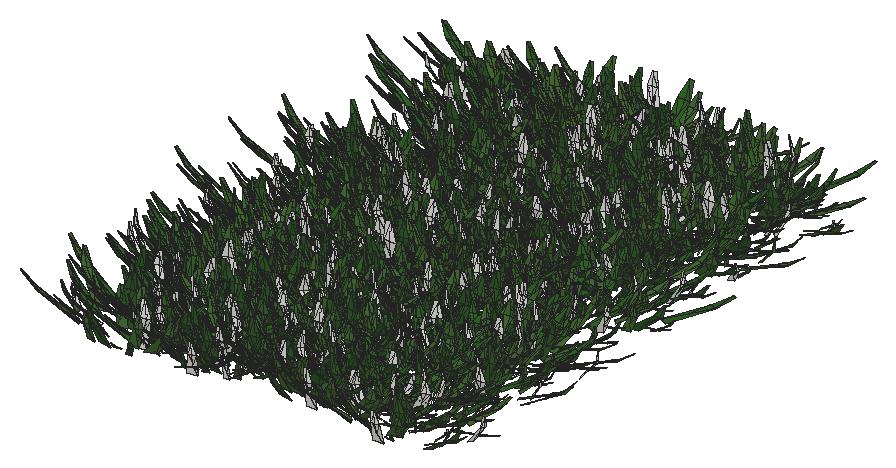
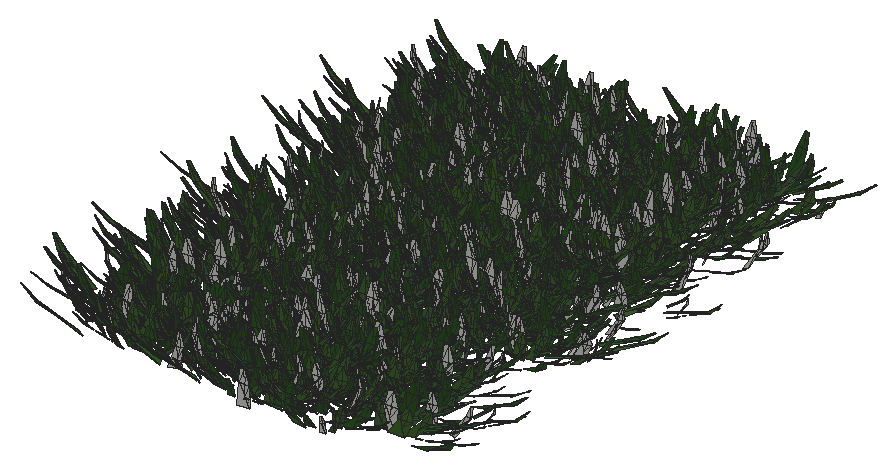
# SketchUp Ruby script. Lengths in inches.
U = 1.inch
M = Sketchup.active_model
def pt(a) = Geom::Point3d.new(a.map { |v| v * U })
def face(e, loops, mat)
  f = e.add_face(loops[0].map { |a| pt(a) })
  loops[1..].each { |l| e.add_face(l.map { |a| pt(a) }).erase! }
  f.material = f.back_material = mat if mat
  f
end
# faces: each face lists its corners as indices into pts; further lists are holes
def faces(e, pts, list, mat = nil) = list.each { |f| face(e, (f[0].is_a?(Array) ? f : [f]).map { |l| l.map { |i| pts[i] } }, mat) }
# xy, xz, yz: faces in a plane at the given z, y or x. An outline is a flat list of corners, or four numbers for a rectangle; further outlines are holes
def ring(l) = l.size == 4 ? [[l[0], l[1]], [l[2], l[1]], [l[2], l[3]], [l[0], l[3]]] : l.each_slice(2).to_a
def flat(e, list, mat, &to3) = list.each { |f| face(e, (f[0].is_a?(Array) ? f : [f]).map { |l| ring(l).map { |u, v| to3.(u, v) } }, mat) }
def xy(e, z, list, mat = nil) = flat(e, list, mat) { |x, y| [x, y, z] }
def xz(e, y, list, mat = nil) = flat(e, list, mat) { |x, z| [x, y, z] }
def yz(e, x, list, mat = nil) = flat(e, list, mat) { |y, z| [x, y, z] }
def lines(e, pts, list) = list.each { |a, b| e.add_line(pt(pts[a]), pt(pts[b])) }
# prism: a flat outline (further loops are holes) pulled along v
def prism(e, loops, v, mat = nil)
  f = face(e, loops, mat); d = Geom::Vector3d.new(v.map { |x| x * U })
  f.pushpull(f.normal.samedirection?(d) ? d.length : -d.length)
end
def box(e, o, s, mat = nil) = prism(e, [[o, [o[0] + s[0], o[1], o[2]], [o[0] + s[0], o[1] + s[1], o[2]], [o[0], o[1] + s[1], o[2]]]], [0, 0, s[2]], mat)
def at(x, y, z, deg = 0) = Geom::Transformation.translation(pt([x, y, z])) * Geom::Transformation.rotation(ORIGIN, Z_AXIS, deg.degrees)
def axes(o, x, y, z) = Geom::Transformation.new([*x, 0, *y, 0, *z, 0, *pt(o).to_a, 1])
def part(name) = M.definitions.add(name)
# library, detail: a bought-in or finely detailed component or shape, given as its bounding box
def library(name, o, s) = part(name).tap { |d| box(d.entities, o, s) }
def detail(e, o, s) = box(e.add_group.entities, o, s)
def put(e, d, t, mat = nil) = e.add_instance(d, t).tap { |i| i.material = mat if mat }
def group(e, t, mat = nil) = e.add_group.tap { |g| g.transformation = t; g.material = mat if mat }.entities
root = M.entities
M.materials.add("Material82").color = [68, 110, 58]
M.materials.add("Material83").color = [48, 90, 38]
M.materials.add("Material84").color = [68, 110, 48]
M.materials.add("Material85").color = [48, 90, 48]
M.materials.add("Material86").color = [58, 110, 58]
M.materials.add("Material87").color = [58, 90, 38]
M.materials.add("Material88").color = [68, 100, 58]
M.materials.add("Material89").color = [48, 100, 38]
c1 = part("grass00")
p = [[-0.6875,0.15,0],[-0.56,0.08,5.52],[-0.04,0.03,2.76],[0.48,-0.02,0],[0.35,-0.02,5.52],[-0.1,-0.14,5.52],
  [-0.12,0.65,8.37],[-0.42,0.65,8.37]]
faces(c1.entities,p,[[0,1,2,3],[3,2,4],[1,5,2],[5,4,2],[1,6,5],[4,5,6],[7,6,1]])
c2 = part("Group16\#1")
put(c2.entities,c1,axes([1.44,-0.61,-0.01],[0.05352,0.12609,0],[-0.10704,0.04543,0.07239],[0.06664,-0.02828,0.11628]),"Material85")
put(c2.entities,c1,axes([0.76,-0.15,-0.01],[0.04676,0.24062,0],[-0.23162,0.04501,0.06642],[0.0652,-0.01267,0.23595]),"Material82")
put(c2.entities,c1,axes([0.79,0.01,-0.01],[-0.00606,0.34651,0],[-0.34381,-0.00602,0.0432],[0.04319,0.00076,0.34386]))
put(c2.entities,c1,axes([1,0.23,-0.01],[-0.07192,0.31144,0],[-0.28722,-0.06632,0.1236],[0.12043,0.02781,0.29478]),"Material84")
put(c2.entities,c1,axes([1.66,0.77,-0.01],[-0.13828,0.29651,0],[-0.21551,-0.1005,0.22471],[0.20365,0.09498,0.23779]),"Material89")
put(c2.entities,c1,axes([0.6875,0.52,-0.01],[-0.18126,0.24051,0],[-0.22746,-0.17142,0.09788],[0.07817,0.05891,0.28481]),"Material84")
put(c2.entities,c1,axes([0.68,0.78,-0.01],[-0.215,0.18688,0],[-0.12385,-0.14248,0.21334],[0.13995,0.16101,0.18878]),"Material82")
put(c2.entities,c1,axes([0.56,1,-0.01],[-0.13756,0.07624,0],[-0.06159,-0.11112,0.0927],[0.04494,0.08108,0.12705]),"Material84")
put(c2.entities,c1,axes([0.2,0.64,-0.01],[-0.23729,0.07254,0],[-0.05711,-0.18681,0.153],[0.04473,0.14632,0.19535]),"Material89")
put(c2.entities,c1,axes([0.0625,0.72,-0.01],[-0.28874,0.02525,0],[-0.02179,-0.24916,0.14647],[0.01276,0.14591,0.25012]),"Material82")
put(c2.entities,c1,axes([-0.08,0.62,-0.01],[-0.34089,-0.04187,0],[0.03255,-0.26504,0.216],[-0.02633,0.21439,0.26703]),"Material89")
put(c2.entities,c1,axes([-0.34,0.98,-0.01],[-0.14314,-0.0493,0],[0.04397,-0.12769,0.06843],[-0.02228,0.0647,0.13505]),"Material89")
put(c2.entities,c1,axes([-0.87,1.45,-0.01],[-0.23488,-0.14114,0],[0.13761,-0.22901,0.06087],[-0.03135,0.05217,0.26717]))
put(c2.entities,c1,axes([-0.72,0.77,-0.01],[-0.14208,-0.13251,0],[0.07209,-0.0773,0.16301],[-0.11118,0.11922,0.1057]),"Material89")
put(c2.entities,c1,axes([-0.62,0.43,-0.01],[-0.14845,-0.21203,0],[0.18654,-0.13061,0.12304],[-0.10079,0.07057,0.22772]),"Material82")
put(c2.entities,c1,axes([-0.68,0.29,-0.01],[-0.13639,-0.32136,0],[0.31723,-0.13464,0.05579],[-0.05136,0.0218,0.34462]),"Material83")
put(c2.entities,c1,axes([-0.64,0.125,-0.01],[-0.0458,-0.23569,0],[0.22124,-0.043,0.08276],[-0.08124,0.01579,0.22538]),"Material86")
put(c2.entities,c1,axes([-1.6,-0.03,-0.01],[0.00576,-0.32897,0],[0.27526,0.00482,0.18018],[-0.18015,-0.00315,0.2753]),"Material84")
put(c2.entities,c1,axes([-1.36,-0.31,-0.01],[0.05718,-0.24765,0],[0.18172,0.04196,0.17267],[-0.16825,-0.03885,0.1865]),"Material89")
put(c2.entities,c1,axes([-1.54,-0.72,-0.01],[0.06537,-0.14017,0],[0.13555,0.06321,0.03939],[-0.0357,-0.01665,0.14956]))
put(c2.entities,c1,axes([-1.19,-0.9,-0.01],[0.09597,-0.12735,0],[0.11214,0.08451,0.07557],[-0.06035,-0.04548,0.14042]),"Material88")
put(c2.entities,c1,axes([-0.47,-0.54,-0.01],[0.11588,-0.10072,0],[0.0618,0.0711,0.12124],[-0.07953,-0.0915,0.0942]))
put(c2.entities,c1,axes([-0.47,-0.84,-0.01],[0.11927,-0.0661,0],[0.06603,0.11913,0.00646],[-0.00313,-0.00565,0.13621]),"Material84")
put(c2.entities,c1,axes([-0.38,-1.24,-0.01],[0.28037,-0.08571,0],[0.0618,0.20215,0.20315],[-0.05939,-0.19428,0.21139]),"Material88")
put(c2.entities,c1,axes([-0.06,-0.66,-0.01],[0.22719,-0.01987,0],[0.01247,0.14255,0.17758],[-0.01547,-0.17691,0.1431]),"Material87")
put(c2.entities,c1,axes([0.11,-0.89,-0.01],[0.14882,0.01828,0],[-0.01058,0.08611,0.12229],[0.01491,-0.12138,0.08676]),"Material85")
put(c2.entities,c1,axes([0.25,-0.72,-0.01],[0.20481,0.07053,0],[-0.06206,0.18022,0.10291],[0.03351,-0.0973,0.1906]),"Material85")
put(c2.entities,c1,axes([0.85,-1.42,-0.01],[0.16481,0.09904,0],[-0.09472,0.15762,0.05616],[0.02893,-0.04814,0.18389]),"Material84")
put(c2.entities,c1,axes([1.01,-1.09,-0.01],[0.21858,0.20385,0],[-0.17495,0.1876,0.15339],[0.10462,-0.11218,0.25652]),"Material89")
put(c2.entities,c1,axes([1.01,-0.71,-0.01],[0.08733,0.12473,0],[-0.06445,0.04512,0.13037],[0.1068,-0.07477,0.07867]),"Material85")
c3 = part("Group15\#1")
put(c3.entities,c2,at(0,0,0))
c4 = part("3darcstudiotree_grass00\#1")
put(c4.entities,c3,at(0,0,0))
put(root,c4,axes([1826.71,976.55,-29.74],[-0.54088,1.62044,0],[-3.31155,-0.17191,-0.03263],[-0.19335,-0.01004,1.49628]))
put(root,c4,axes([1826.9,975.01,-29.74],[3.70566,-0.42814,0],[1.15173,1.5504,-0.01036],[0.01836,0.02471,1.93559]))
put(root,c4,axes([1827.4,940.33,-29.74],[2.92691,-1.3802,0],[3.11862,1.02859,-0.02296],[0.10607,0.03499,1.8355]))
put(root,c4,axes([1827.2,994.31,-29.74],[-0.97344,1.33602,0],[-4.5066,-0.51069,-0.06106],[-0.24596,-0.02787,1.47293]))
put(root,c4,axes([1827.02,963.53,-29.74],[4.64499,-0.27977,0],[0.53132,1.372,-0.02943],[0.02555,0.06597,1.51666]))
put(root,c4,axes([1828.48,961.14,-29.74],[-0.18207,-1.50592,0],[4.09357,-0.07698,-0.05646],[0.28834,-0.00542,1.57058]))
put(root,c4,axes([1827.15,950.76,-29.74],[2.47814,1.17598,0],[-3.14029,1.02922,-0.05468],[-0.21842,0.07159,1.58958]))
put(root,c4,axes([1827.12,973.05,-29.74],[4.42055,0.62646,0],[-1.4719,1.61538,-0.03831],[-0.06085,0.06679,1.53223]))
put(root,c4,axes([1827.64,989.9,-29.74],[4.51641,-0.1704,0],[0.33815,1.39393,-0.00501],[0.00291,0.012,1.62495]))
put(root,c4,axes([1827.34,952.9375,-29.74],[2.33395,1.59128,0],[-3.69314,0.84246,-0.02506],[-0.12399,0.02828,1.82822]))
put(root,c4,axes([1827.93,944.71,-29.74],[3.72841,-0.11021,0],[0.34874,1.83494,-0.00347],[0.00143,0.00753,1.92949]))
put(root,c4,axes([1828.92,986.01,-29.74],[-2.15234,1.14546,0],[-3.3995,-0.99347,-0.05517],[-0.2418,-0.07066,1.72999]))
put(root,c4,axes([1828.23,959.73,-29.74],[2.3917,1.38211,0],[-2.775,0.74686,-0.01403],[-0.09111,0.02452,1.97952]))
put(root,c4,axes([1828.32,968.4,-29.74],[3.05644,0.96272,0],[-2.54771,1.25799,-0.04015],[-0.1144,0.05649,1.39698]))
put(root,c4,axes([1828.88,955.42,-29.74],[0.44258,1.4547,0],[-3.4051,0.16112,-0.01784],[-0.12417,0.00588,1.80168]))
put(root,c4,axes([1830.52,982.97,-29.74],[-1.45799,-1.43911,0],[3.11235,-0.49041,-0.01431],[0.09188,-0.01448,1.73701]))
put(root,c4,axes([1830.67,942.56,-29.74],[-2.77273,1.25915,0],[-2.61353,-0.89509,-0.01448],[-0.05898,-0.0202,1.39954]))
put(root,c4,axes([1831.64,944.09,-29.74],[-3.67224,-0.62774,0],[1.3268,-1.20717,-0.04544],[0.10775,-0.09803,1.4908]))
put(root,c4,axes([1831.89,976.69,-29.74],[-4.47177,0.4092,0],[-0.80597,-1.36984,-0.03599],[-0.04373,-0.07433,1.43677]))
put(root,c4,axes([1831.27,954.99,-29.74],[-3.07968,1.30519,0],[-3.32937,-1.22181,-0.01383],[-0.04412,-0.01619,1.48532]))
put(root,c4,axes([1830.8125,966.41,-29.74],[3.91717,0.58785,0],[-1.40512,1.45623,-0.01203],[-0.02325,0.0241,1.60927]))
put(root,c4,axes([1832.68,961.55,-29.74],[-1.04981,-1.26066,0],[3.51989,-0.45588,-0.02104],[0.10484,-0.01358,1.45661]))
put(root,c4,axes([1831.94,958.11,-29.74],[3.15172,-0.92963,0],[2.70365,1.42561,-0.02614],[0.06865,0.0362,1.48366]))
put(root,c4,axes([1832.72,964.35,-29.74],[-4.56421,0.17831,0],[-0.33265,-1.32435,-0.0174],[-0.0117,-0.04658,1.72585]))
put(root,c4,axes([1833.2,990.04,-29.74],[-3.08784,-0.53374,0],[1.78756,-1.6084,-0.00176],[0.00414,-0.00372,1.95594]))
put(root,c4,axes([1832.26,950.46,-29.74],[-2.14552,1.35971,0],[-3.80804,-0.93454,-0.04897],[-0.2422,-0.05944,1.9584]))
put(root,c4,axes([1831.72,947.17,-29.74],[3.03533,0.518,0],[-1.31858,1.2017,-0.02703],[-0.08286,0.07551,1.9211]))
put(root,c4,axes([1833.56,972.37,-29.74],[-2.79081,-0.68685,0],[2.20267,-1.39196,-0.00523],[0.01654,-0.01045,1.86317]))
put(root,c4,axes([1833.69,975.79,-29.74],[-3.42781,-0.73376,0],[1.91044,-1.38806,-0.04387],[0.11882,-0.08633,1.70431]))
put(root,c4,axes([1833,948.51,-29.74],[-3.41152,0.77464,0],[-2.34689,-1.60751,-0.0199],[-0.0471,-0.03226,1.67187]))
put(root,c4,axes([1832.01,971.16,-29.74],[1.53269,1.16919,0],[-3.90157,0.79546,-0.03477],[-0.15934,0.03249,1.69826]))
put(root,c4,axes([1833.29,959.12,-29.74],[-2.82754,1.11661,0],[-2.90837,-1.14544,-0.05526],[-0.21558,-0.0849,1.69871]))
put(root,c4,axes([1833.3,952.53,-29.74],[2.39859,-1.38317,0],[2.89597,0.78107,-0.02882],[0.1286,0.03468,1.42183]))
put(root,c4,axes([1833.73,996.9375,-29.74],[0.37671,-1.60669,0],[3.58296,0.13066,-0.04487],[0.23434,0.00855,1.41449]))
put(root,c4,axes([1834.14,995.4375,-29.74],[-4.41181,-0.09171,0],[0.23476,-1.75641,-0.0488],[0.01273,-0.09527,1.65721]))
put(root,c4,axes([1834,940.76,-29.74],[-3.47293,0.19496,0],[-0.50842,-1.40863,-0.03826],[-0.03299,-0.09141,1.65468]))
put(root,c4,axes([1834.5625,991.8,-29.74],[-4.2727,-0.29638,0],[0.78575,-1.76178,-0.04722],[0.03378,-0.07573,1.40384]))
put(root,c4,axes([1833.22,987.32,-29.74],[-0.9668,1.66725,0],[-3.92404,-0.3539,-0.0233],[-0.11915,-0.01075,1.58282]))
put(root,c4,axes([1833.27,968.64,-29.74],[3.78841,0.96012,0],[-2.55963,1.5708,-0.03131],[-0.07104,0.04359,1.48921]))
put(root,c4,axes([1833.51,981.64,-29.74],[2.7139,1.45109,0],[-3.63417,1.0571,-0.05484],[-0.17137,0.04985,1.31443]))
put(root,c4,axes([1834.07,979.63,-29.74],[3.41186,0.04199,0],[-0.11049,1.39641,-0.01718],[-0.0038,0.04797,1.88076]))
put(root,c4,axes([1836.15,958.1,-29.74],[-3.09292,-0.92086,0],[2.57207,-1.3436,-0.01411],[0.04505,-0.02353,1.69584]))
put(root,c4,axes([1834.3,985.4,-29.74],[0.1551,1.54916,0],[-4.73746,0.07377,-0.04149],[-0.18002,0.0028,1.54325]))
put(root,c4,axes([1836.33,976.88,-29.74],[0.67498,-1.80639,0],[4.18251,0.24307,-0.00777],[0.03281,0.00191,1.3523]))
put(root,c4,axes([1836.49,972.86,-29.74],[-0.75947,-1.30953,0],[4.19896,-0.37875,-0.04627],[0.26037,-0.02349,1.86363]))
put(root,c4,axes([1836.53,959.17,-29.74],[-4.1346,0.13575,0],[-0.2838,-1.34436,-0.02559],[-0.01617,-0.0766,1.95328]))
put(root,c4,axes([1837.31,970.48,-29.74],[1.00092,-1.32759,0],[4.42574,0.51896,-0.06029],[0.29852,0.035,1.78762]))
put(root,c4,axes([1837,991.66,-29.74],[2.10537,-1.23806,0],[3.71835,0.98344,-0.05795],[0.27877,0.07373,1.94389]))
put(root,c4,axes([1836.35,946.54,-29.74],[3.79547,0.16316,0],[-0.37027,1.33962,-0.03498],[-0.02197,0.07948,1.48455]))
put(root,c4,axes([1837.2,966.05,-29.74],[-3.00276,0.99555,0],[-2.11915,-0.9941,-0.00081],[-0.00373,-0.00175,1.76997]))
put(root,c4,axes([1838.32,984.25,-29.74],[-0.04764,-1.42757,0],[4.50476,-0.02338,-0.00745],[0.04284,-0.00022,1.94284]))
put(root,c4,axes([1837.01,942.28,-29.74],[0.27257,1.5962,0],[-3.57048,0.09483,-0.04154],[-0.28788,0.00765,1.86323]))
put(root,c4,axes([1838.46,979.48,-29.74],[-4.51182,-0.35471,0],[0.87439,-1.72977,-0.01918],[0.02129,-0.04212,1.90358]))
put(root,c4,axes([1837.23,986.4375,-29.74],[2.9902,-0.77103,0],[1.83544,1.10708,-0.045],[0.13449,0.08112,1.37282]))
put(root,c4,axes([1838.51,964.39,-29.74],[0.52861,-1.48035,0],[4.44113,0.24665,-0.00524],[0.03043,0.00169,1.97007]))
put(root,c4,axes([1836.8,953.83,-29.74],[1.62026,1.14881,0],[-2.90984,0.63829,-0.00131],[-0.00892,0.00196,1.9458]))
put(root,c4,axes([1837.83,944.28,-29.74],[-3.07094,0.93295,0],[-2.23562,-1.14452,-0.00087],[-0.00325,-0.00166,1.68429]))
put(root,c4,axes([1838.87,950.63,-29.74],[-1.32818,-1.26932,0],[4.11875,-0.67029,-0.01762],[0.07227,-0.01176,1.48208]))
put(root,c4,axes([1836.96,948.25,-29.74],[3.48613,0.95688,0],[-2.23612,1.26704,-0.01513],[-0.04219,0.02391,1.43215]))
put(root,c4,axes([1838.05,981.34,-29.74],[3.73229,-0.67208,0],[1.78653,1.54305,-0.05401],[0.10032,0.08665,1.44188]))
put(root,c4,axes([1839.69,994.4375,-29.74],[-3.64932,-0.7532,0],[1.94147,-1.463,-0.05348],[0.14522,-0.10943,1.83786]))
put(root,c4,axes([1838.4,968.61,-29.74],[4.39358,-0.14103,0],[0.35283,1.70956,-0.02372],[0.00876,0.04243,1.48337]))
put(root,c4,axes([1839.88,996.02,-29.74],[-4.22243,0.41861,0],[-0.86072,-1.35028,-0.03206],[-0.04838,-0.0759,1.63785]))
put(root,c4,axes([1838.9,987.81,-29.74],[2.4549,0.99675,0],[-3.14112,1.20322,-0.03466],[-0.14383,0.05509,1.89896]))
put(root,c4,axes([1838.95,974.69,-29.74],[3.48474,0.89145,0],[-2.45497,1.49256,-0.05832],[-0.13986,0.08503,1.48992]))
put(root,c4,axes([1839.48,990.48,-29.74],[-0.03901,1.43427,0],[-3.74587,-0.01585,-0.03184],[-0.19446,-0.00082,1.71482]))
put(root,c4,axes([1839.86,962.16,-29.74],[-1.95042,1.47202,0],[-4.16072,-0.85742,-0.06253],[-0.2988,-0.06158,1.89715]))
put(root,c4,axes([1839.76,955.55,-29.74],[3.54296,-0.10072,0],[0.24357,1.33252,-0.00836],[0.00467,0.02557,1.97523]))
put(root,c4,axes([1841.96,972.91,-29.74],[-3.58618,-0.76762,0],[2.12856,-1.54662,-0.04044],[0.10752,-0.07813,1.86421]))
put(root,c4,axes([1842.24,968.36,-29.74],[-3.71376,-0.4791,0],[1.06109,-1.27925,-0.035],[0.07367,-0.08882,1.73222]))
put(root,c4,axes([1842.79,988.51,-29.74],[-3.76687,-0.82913,0],[2.27178,-1.60524,-0.0179],[0.04066,-0.02873,1.62858]))
put(root,c4,axes([1841.95,950.84,-29.74],[-3.28554,0.84585,0],[-2.43757,-1.4726,-0.04574],[-0.1384,-0.08361,1.85022]))
put(root,c4,axes([1842.7,949.5,-29.74],[0.43132,-1.66774,0],[3.95027,0.1589,-0.00761],[0.04938,0.00199,1.94156]))
put(root,c4,axes([1842.96,976.58,-29.74],[-3.03865,-1.23581,0],[2.76731,-1.05827,-0.04714],[0.18592,-0.0711,1.58733]))
put(root,c4,axes([1841.55,945.875,-29.74],[4.71636,-0.1967,0],[0.48906,1.82382,-0.02611],[0.01545,0.05763,1.96192]))
put(root,c4,axes([1842.64,979.12,-29.74],[-3.07129,1.23004,0],[-2.90171,-1.12685,-0.02428],[-0.07533,-0.02925,1.32917]))
put(root,c4,axes([1843.55,953.86,-29.74],[-3.14124,-0.52931,0],[1.80451,-1.66556,-0.04539],[0.09971,-0.09203,1.92461]))
put(root,c4,axes([1842.27,997.4,-29.74],[4.37264,-0.16186,0],[0.38997,1.63854,-0.03728],[0.02119,0.08905,1.90298]))
put(root,c4,axes([1842.62,991.83,-29.74],[4.22982,-0.69798,0],[1.45654,1.37281,-0.04818],[0.09708,0.0915,1.47658]))
put(root,c4,axes([1842.875,990.87,-29.74],[3.5272,-0.10967,0],[0.36977,1.84972,-0.03935],[0.01267,0.0634,1.44542]))
put(root,c4,axes([1843.61,983.14,-29.74],[2.22522,-0.98382,0],[3.26699,1.14926,-0.04874],[0.15967,0.05617,1.44038]))
put(root,c4,axes([1842.81,957.58,-29.74],[4.40761,-0.00182,0],[0.00468,1.76466,-0.04894],[0.00022,0.08123,1.41164]))
put(root,c4,axes([1844.71,975.77,-29.74],[-3.1255,-0.93872,0],[2.35839,-1.22127,-0.01582],[0.04515,-0.02338,1.37394]))
put(root,c4,axes([1843.66,971.33,-29.74],[-2.15998,1.50569,0],[-3.5128,-0.78375,-0.02589],[-0.10439,-0.02329,1.40149]))
put(root,c4,axes([1844.14,994.6875,-29.74],[2.50422,-1.12718,0],[2.64209,0.91293,-0.00209],[0.0092,0.00318,1.54397]))
put(root,c4,axes([1844.3,986.33,-29.74],[-3.79899,1.04858,0],[-2.13311,-1.20197,-0.01309],[-0.05055,-0.02848,1.87779]))
put(root,c4,axes([1844.97,956.11,-29.74],[-0.77442,-1.59147,0],[3.42237,-0.25901,-0.00431],[0.02185,-0.00165,1.34772]))
put(root,c4,axes([1845.25,942.86,-29.74],[-1.56215,-1.16443,0],[3.47638,-0.72535,-0.0302],[0.1517,-0.03165,1.67548]))
put(root,c4,axes([1845.33,961.6,-29.74],[0.16922,-1.40325,0],[3.56749,0.06691,-0.0123],[0.08099,0.00152,1.7643]))
put(root,c4,axes([1844.16,965.91,-29.74],[3.21803,0.34517,0],[-1.06694,1.54707,-0.02379],[-0.03071,0.04453,1.49895]))
put(root,c4,axes([1843.92,959.62,-29.74],[1.18275,1.22871,0],[-4.35683,0.65227,-0.02635],[-0.11985,0.01794,1.69955]))
put(root,c4,axes([1845.58,981.5,-29.74],[-4.55654,0.30056,0],[-0.72952,-1.72007,-0.00717],[-0.00538,-0.01268,1.50735]))
put(root,c4,axes([1845.07,964.58,-29.74],[2.66801,-0.76193,0],[2.24823,1.2244,-0.04376],[0.15596,0.08494,1.7457]))
put(root,c4,axes([1847.17,972.15,-29.74],[-2.4386,-1.43306,0],[3.07254,-0.81318,-0.00883],[0.05033,-0.01332,1.90461]))
put(root,c4,axes([1847.54,990.58,-29.74],[-2.69612,-1.17454,0],[3.29179,-1.17522,-0.01753],[0.05781,-0.02064,1.48083]))
put(root,c4,axes([1845.5,944.46,-29.74],[-0.169,1.77802,0],[-4.32571,-0.06395,-0.00219],[-0.00941,-0.00014,1.39308]))
put(root,c4,axes([1847.73,948.11,-29.74],[-3.83813,-1.06248,0],[2.06139,-1.15817,-0.02484],[0.08815,-0.04953,1.66133]))
put(root,c4,axes([1847.43,984.43,-29.74],[-4.08007,0.11151,0],[-0.22831,-1.29918,-0.01842],[-0.00694,-0.03947,1.34789]))
put(root,c4,axes([1847.91,942.67,-29.74],[-3.13096,0.65051,0],[-1.62991,-1.22011,-0.01732],[-0.0588,-0.04402,1.90951]))
put(root,c4,axes([1849.12,995.01,-29.74],[-1.34356,-1.54381,0],[4.22745,-0.57221,-0.00214],[0.01038,-0.00141,1.72072]))
put(root,c4,axes([1847.18,950.22,-29.74],[3.83567,0.80348,0],[-1.71741,1.27513,-0.04207],[-0.13622,0.10114,1.89419]))
put(root,c4,axes([1847.6,966.3125,-29.74],[2.14752,1.24419,0],[-2.84206,0.76295,-0.02533],[-0.12904,0.03464,1.58831]))
put(root,c4,axes([1848.2,988.64,-29.74],[4.00755,-0.76372,0],[1.77132,1.44561,-0.00312],[0.00773,0.00631,1.73901]))
put(root,c4,axes([1847.9,959.82,-29.74],[0.92286,1.78615,0],[-4.03148,0.32396,-0.0503],[-0.25163,0.02022,1.57458]))
put(root,c4,axes([1848.24,974.88,-29.74],[-1.5079,1.48015,0],[-3.78766,-0.60014,-0.02547],[-0.10708,-0.01697,1.38631]))
put(root,c4,axes([1849.28,956.86,-29.74],[0.88426,-1.72062,0],[4.38154,0.35021,-0.041],[0.21175,0.01693,1.76588]))
put(root,c4,axes([1848.11,952.75,-29.74],[4.1439,0.48612,0],[-1.21296,1.60815,-0.03162],[-0.038,0.05038,1.3441]))
put(root,c4,axes([1847.97,967.88,-29.74],[2.12924,1.06786,0],[-3.55371,1.10206,-0.01217],[-0.05143,0.01595,1.82194]))
put(root,c4,axes([1849.54,943.78,-29.74],[1.5808,-1.43275,0],[3.65536,0.62726,-0.04597],[0.19603,0.03364,1.38947]))
put(root,c4,axes([1850.43,947.09,-29.74],[-4.27451,-0.64112,0],[1.27307,-1.32012,-0.04106],[0.09351,-0.09696,1.71966]))
put(root,c4,axes([1850.35,992.01,-29.74],[-3.75297,0.08152,0],[-0.23562,-1.68719,-0.02509],[-0.00578,-0.04142,1.34616]))
put(root,c4,axes([1851,982.35,-29.74],[-0.74737,-1.75822,0],[4.00395,-0.2647,-0.02808],[0.1526,-0.01009,1.67665]))
put(root,c4,axes([1850.24,963.58,-29.74],[2.37533,-1.57622,0],[3.03149,0.71052,-0.0411],[0.20378,0.04776,1.52451]))
put(root,c4,axes([1849.44,977.06,-29.74],[3.22242,0.46316,0],[-1.61234,1.7447,-0.03532],[-0.06153,0.06658,1.79519]))
put(root,c4,axes([1849.93,971.43,-29.74],[0.53134,1.4221,0],[-3.42638,0.19911,-0.04131],[-0.21204,0.01232,1.34689]))
put(root,c4,axes([1850.41,962.64,-29.74],[3.9417,-1.03975,0],[1.84996,1.09076,-0.03191],[0.12762,0.07525,1.79443]))
put(root,c4,axes([1850.8,955.36,-29.74],[3.56947,-0.45549,0],[1.31887,1.60745,-0.01717],[0.02449,0.02985,1.48777]))
put(root,c4,axes([1850.88,978.75,-29.74],[0.55525,1.71346,0],[-3.482,0.17549,-0.04145],[-0.30813,0.01553,1.97198]))
put(root,c4,axes([1850.63,985.74,-29.74],[3.66484,0.89609,0],[-2.00603,1.27601,-0.03504],[-0.12347,0.07854,1.90819]))
put(root,c4,axes([1852.84,948.68,-29.74],[-1.10349,-1.4395,0],[4.41957,-0.52692,-0.03772],[0.14279,-0.01702,1.36861]))
put(root,c4,axes([1852.64,978.59,-29.74],[-2.20687,1.14075,0],[-3.09016,-0.92978,-0.05103],[-0.23957,-0.07208,1.72023]))
put(root,c4,axes([1853.1,990.62,-29.74],[-3.32366,1.12138,0],[-2.70082,-1.24501,-0.05065],[-0.15287,-0.07047,1.44592]))
put(root,c4,axes([1854.1875,975.37,-29.74],[-2.7638,-1.30283,0],[3.13183,-1.03331,-0.01878],[0.07913,-0.02611,1.68146]))
put(root,c4,axes([1854.41,968.09,-29.74],[-3.16827,-0.67396,0],[1.62868,-1.19079,-0.04409],[0.1208,-0.08832,1.48398]))
put(root,c4,axes([1854.17,976.43,-29.74],[-4.1698,0.79339,0],[-1.666,-1.36181,-0.02532],[-0.06287,-0.05139,1.64221]))
put(root,c4,axes([1853.13,996.75,-29.74],[3.81533,0.48086,0],[-1.13696,1.40304,-0.03842],[-0.0798,0.09848,1.90991]))
put(root,c4,axes([1853.74,961.15,-29.74],[3.77642,-0.7823,0],[1.66108,1.24712,-0.02304],[0.07142,0.05362,1.78453]))
put(root,c4,axes([1855.27,988.36,-29.74],[0.63263,-1.77026,0],[4.09912,0.22783,-0.02402],[0.14113,0.00784,1.84088]))
put(root,c4,axes([1855.41,952.63,-29.74],[-4.44839,0.03138,0],[-0.07411,-1.6342,-0.01042],[-0.00109,-0.02408,1.82123]))
put(root,c4,axes([1855.4,941.76,-29.74],[-3.4085,0.44598,0],[-1.18576,-1.40948,-0.04681],[-0.08042,-0.0956,1.53984]))
put(root,c4,axes([1854.15,951.4,-29.74],[3.54482,0.3991,0],[-1.20365,1.66273,-0.00872],[-0.01104,0.01525,1.51538]))
put(root,c4,axes([1854.78,981.39,-29.74],[-0.28998,1.73456,0],[-3.34694,-0.08702,-0.03816],[-0.29536,-0.00768,1.95014]))
put(root,c4,axes([1854,946.2,-29.74],[3.41397,1.21641,0],[-2.3032,1.00536,-0.00582],[-0.0237,0.01035,1.56404]))
put(root,c4,axes([1854.125,957.63,-29.74],[2.93721,1.2592,0],[-3.10849,1.12772,-0.033],[-0.144,0.05224,1.87715]))
put(root,c4,axes([1856.29,959.2,-29.74],[-1.1478,-1.40641,0],[4.093,-0.51953,-0.0477],[0.19511,-0.02477,1.385]))
put(root,c4,axes([1856.68,945.06,-29.74],[-2.49924,-1.08664,0],[2.82442,-1.01033,-0.0539],[0.19999,-0.07154,1.43163]))
put(root,c4,axes([1855.07,964.59,-29.74],[2.93445,0.88211,0],[-2.13254,1.10335,-0.01463],[-0.05848,0.03025,1.73802]))
put(root,c4,axes([1855.1875,956.09,-29.74],[3.48566,0.55514,0],[-1.55719,1.52067,-0.03343],[-0.07577,0.07399,1.88641]))
put(root,c4,axes([1855.65,994.63,-29.74],[-0.15322,1.4871,0],[-3.57108,-0.05722,-0.03031],[-0.19833,-0.00318,1.75443]))
put(root,c4,axes([1855.35,973.48,-29.74],[3.31433,0.47754,0],[-1.51472,1.63504,-0.04863],[-0.07862,0.08486,1.5585]))
put(root,c4,axes([1856.58,993.22,-29.74],[-3.94658,0.83198,0],[-2.08533,-1.53849,-0.02635],[-0.05206,-0.03841,1.3895]))
put(root,c4,axes([1855.19,985.74,-29.74],[2.20824,1.44568,0],[-4.06639,0.96604,-0.01693],[-0.06521,0.01549,1.59984]))
put(root,c4,axes([1855.93,970.04,-29.74],[4.53975,0.53985,0],[-1.08694,1.4216,-0.04516],[-0.08333,0.10898,1.80387]))
put(root,c4,axes([1856.64,982.97,-29.74],[-2.27595,1.46975,0],[-3.85308,-0.92798,-0.0342],[-0.14118,-0.034,1.63693]))
